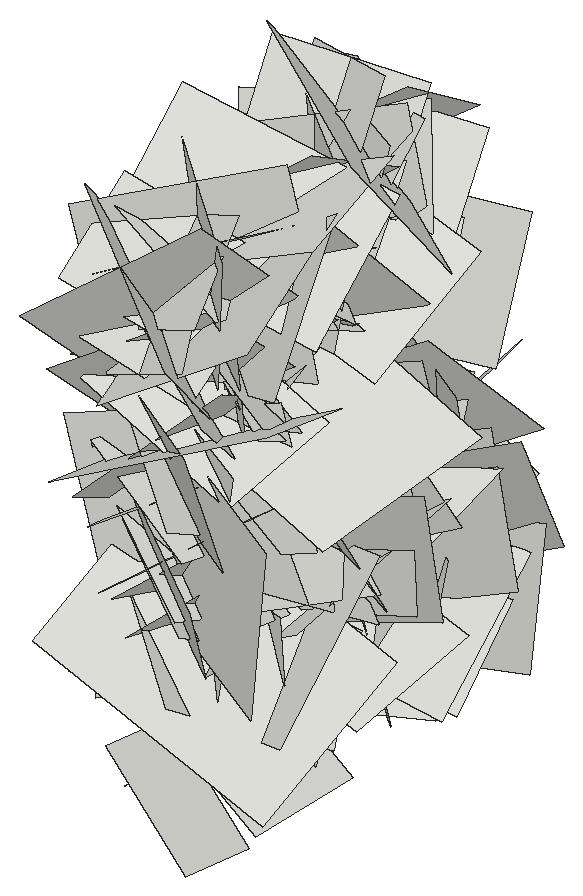
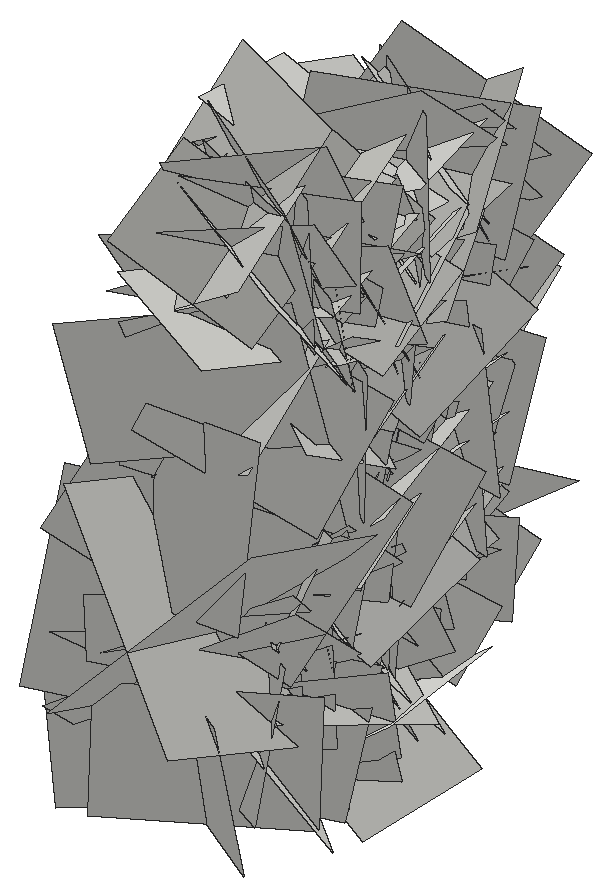
# SketchUp Ruby script. Lengths in inches.
U = 1.inch
M = Sketchup.active_model
def pt(a) = Geom::Point3d.new(a.map { |v| v * U })
def face(e, loops, mat)
  f = e.add_face(loops[0].map { |a| pt(a) })
  loops[1..].each { |l| e.add_face(l.map { |a| pt(a) }).erase! }
  f.material = f.back_material = mat if mat
  f
end
# faces: each face lists its corners as indices into pts; further lists are holes
def faces(e, pts, list, mat = nil) = list.each { |f| face(e, (f[0].is_a?(Array) ? f : [f]).map { |l| l.map { |i| pts[i] } }, mat) }
# xy, xz, yz: faces in a plane at the given z, y or x. An outline is a flat list of corners, or four numbers for a rectangle; further outlines are holes
def ring(l) = l.size == 4 ? [[l[0], l[1]], [l[2], l[1]], [l[2], l[3]], [l[0], l[3]]] : l.each_slice(2).to_a
def flat(e, list, mat, &to3) = list.each { |f| face(e, (f[0].is_a?(Array) ? f : [f]).map { |l| ring(l).map { |u, v| to3.(u, v) } }, mat) }
def xy(e, z, list, mat = nil) = flat(e, list, mat) { |x, y| [x, y, z] }
def xz(e, y, list, mat = nil) = flat(e, list, mat) { |x, z| [x, y, z] }
def yz(e, x, list, mat = nil) = flat(e, list, mat) { |y, z| [x, y, z] }
def lines(e, pts, list) = list.each { |a, b| e.add_line(pt(pts[a]), pt(pts[b])) }
# prism: a flat outline (further loops are holes) pulled along v
def prism(e, loops, v, mat = nil)
  f = face(e, loops, mat); d = Geom::Vector3d.new(v.map { |x| x * U })
  f.pushpull(f.normal.samedirection?(d) ? d.length : -d.length)
end
def box(e, o, s, mat = nil) = prism(e, [[o, [o[0] + s[0], o[1], o[2]], [o[0] + s[0], o[1] + s[1], o[2]], [o[0], o[1] + s[1], o[2]]]], [0, 0, s[2]], mat)
def at(x, y, z, deg = 0) = Geom::Transformation.translation(pt([x, y, z])) * Geom::Transformation.rotation(ORIGIN, Z_AXIS, deg.degrees)
def axes(o, x, y, z) = Geom::Transformation.new([*x, 0, *y, 0, *z, 0, *pt(o).to_a, 1])
def part(name) = M.definitions.add(name)
# library, detail: a bought-in or finely detailed component or shape, given as its bounding box
def library(name, o, s) = part(name).tap { |d| box(d.entities, o, s) }
def detail(e, o, s) = box(e.add_group.entities, o, s)
def put(e, d, t, mat = nil) = e.add_instance(d, t).tap { |i| i.material = mat if mat }
def group(e, t, mat = nil) = e.add_group.tap { |g| g.transformation = t; g.material = mat if mat }.entities
root = M.entities
c1 = part("Component\#6")
p = [[0.01,0,0],[0,3.24,4.54],[4.32,3.24,4.54],[4.33,0,0]]
faces(c1.entities,p,[[0,1,2,3]])
put(root,c1,axes([420.52,193.25,29.42],[-0.0602,0.67546,-0.3863],[-0.10598,-0.39045,-0.66802],[0.81797,-0.00088,-0.11498]))
put(root,c1,axes([420.52,194.71,36.49],[-0.01491,0.71707,-0.22931],[-0.11795,-0.22881,-0.70868],[0.78925,-0.02064,-0.11024]))
put(root,c1,axes([424.49,198.67,35.61],[0.10111,0.59855,0.78971],[-0.15679,0.79307,-0.58323],[-1.03859,-0.06146,0.16492]))
put(root,c1,axes([424.49,206.72,25.52],[0.07134,-1.27871,-0.42932],[0.37284,-0.39835,1.24159],[-1.38032,-0.17369,0.31318]))
put(root,c1,axes([424.49,196.41,37.05],[-0.02372,0.78814,-0.36288],[-0.15491,-0.36124,-0.77556],[-0.90659,0.0411,0.14202]))
put(root,c1,axes([424.49,200.08,36.17],[-0.04967,-0.3024,-0.77978],[-0.15753,-0.76557,0.30582],[-0.87244,0.15545,-0.01082]))
put(root,c1,axes([420.52,194.0625,27.88],[-0.03826,-0.32146,0.75655],[-0.14724,0.74878,0.31153],[0.85881,0.11405,0.08712]))
put(root,c1,axes([420.52,192.62,23.41],[-0.0945,0.05137,0.75973],[0.00531,0.76494,-0.05113],[0.80713,0.00098,0.08928]))
put(root,c1,axes([420.52,194.1,30.97],[-0.07757,0.18705,0.69229],[0.05179,0.69557,-0.18277],[0.75837,-0.02837,0.08329]))
put(root,c1,axes([424.49,192.76,27.5],[0.21382,-0.08753,1.03604],[-0.20559,1.03367,0.1251],[-1.08277,-0.21355,0.18084]))
put(root,c1,axes([420.52,197.11,20.7],[-0.0234,0.20043,0.60552],[0.11848,0.59772,-0.19378],[0.66563,-0.09934,0.05578]))
put(root,c1,axes([424.49,194.12,36.42],[0.16155,0.92195,-0.51802],[-0.06641,-0.51458,-0.93426],[-1.119,0.16364,-0.01934]))
put(root,c1,axes([420.52,192.68,25.51],[0.10584,0.56729,0.32604],[-0.07365,0.33715,-0.56532],[0.68964,-0.05105,-0.11041]))
put(root,c1,axes([424.49,198.72,19.65],[0.06387,-1.04135,0.05905],[0.06023,0.06234,1.04135],[-1.10396,-0.05685,0.06023]))
put(root,c1,axes([424.49,194.92,22.54],[-0.07164,-0.895,0.57486],[0.24411,0.55005,0.88344],[-1.1008,0.18023,0.15849]))
put(root,c1,axes([424.49,200.17,25.9],[-0.12286,-0.34825,-0.84521],[0.12526,-0.85054,0.33424],[-0.96086,-0.06635,0.15165]))
put(root,c1,axes([420.52,196.5,26.6],[-0.00001,0.64808,0.59207],[-0.20568,0.57742,-0.63205],[0.90746,0.13088,-0.14325]))
put(root,c1,axes([424.49,195.45,23.05],[-0.08121,0.42866,0.62692],[-0.16296,0.6083,-0.43472],[-0.78836,-0.1699,0.02528]))
put(root,c1,axes([420.52,201.07,39.9375],[-0.03161,0.68058,-0.41337],[-0.06223,-0.41441,-0.67806],[0.84176,-0.00508,-0.06565]))
put(root,c1,axes([420.52,199.74,34.07],[0.11183,-0.60219,-0.2199],[-0.02555,-0.22643,0.6085],[0.67907,0.09065,0.0591]))
put(root,c1,axes([424.49,195.7,29.31],[0.12944,0.87645,-0.3909],[-0.13192,-0.37627,-0.88251],[-1.00866,0.16168,0.06525]))
put(root,c1,axes([424.49,195.4,26.27],[-0.15303,-0.80886,0.21466],[0.08059,0.20425,0.82078],[-0.8834,0.15875,0.0377]))
put(root,c1,axes([420.52,197.17,21.41],[-0.31691,0.51794,0.91951],[-0.05422,0.94746,-0.55031],[1.11735,0.19287,0.23409]))
put(root,c1,axes([424.49,204.82,25.65],[0.12938,-0.11687,-1.00907],[-0.02351,-1.01639,0.11504],[-1.07651,0.00815,-0.12379]))
put(root,c1,axes([420.52,192.15,39.48],[-0.21361,0.71392,-0.72381],[-0.12034,-0.74908,-0.70723],[1.07091,0.05823,-0.22384]))
put(root,c1,axes([424.49,200.1,34.99],[-0.01875,0.74709,-0.59948],[0.09315,-0.59579,-0.74508],[-1.01106,-0.06874,-0.05753]))
put(root,c1,axes([420.52,198.57,33.25],[-0.09717,0.14422,-0.89801],[-0.11089,-0.89824,-0.13357],[0.95769,-0.08937,-0.10658]))
put(root,c1,axes([424.49,201.91,26.14],[0.02369,0.31708,-0.9382],[0.09459,-0.93526,-0.31396],[-1.04548,-0.07743,-0.04967]))
put(root,c1,axes([424.49,195.16,37.28],[-0.08536,-0.54597,-0.55526],[-0.06407,-0.55215,0.55168],[-0.82294,0.09962,0.01464]))
put(root,c1,axes([420.52,196.95,39.61],[-0.06663,0.78722,-0.39485],[-0.0883,-0.3994,-0.78302],[0.92935,0.01849,-0.10271]))
put(root,c1,axes([420.52,194.17,31.15],[-0.1572,-0.65225,0.62778],[-0.00257,0.63643,0.66066],[0.9596,-0.10514,0.10461]))
put(root,c1,axes([424.49,197.53,26.62],[-0.11622,-0.11144,-0.6986],[-0.08861,-0.69994,0.12478],[-0.74462,0.10068,0.09418]))
put(root,c1,axes([424.49,195.33,34.42],[-0.12228,0.30682,0.85432],[0.19875,0.85067,-0.2802],[-0.94146,0.13973,-0.17012]))
put(root,c1,axes([420.52,195.89,35.57],[-0.03273,-0.74668,0.19464],[0.06894,0.19158,0.74527],[0.81502,-0.04619,-0.05522]))
put(root,c1,axes([420.52,192.38,31.46],[0.05244,0.73173,-0.11131],[0.01157,-0.11227,-0.73318],[0.78447,-0.04726,0.01825]))
put(root,c1,axes([424.49,198.41,25.5],[0.14641,-1.02966,0.26735],[0.10928,0.28128,1.03005],[-1.12233,-0.10694,0.13517]))
put(root,c1,axes([424.49,198.86,35.2],[0.14047,0.16017,0.87964],[-0.13868,0.88315,-0.1411],[-0.93754,-0.10664,0.15267]))
put(root,c1,axes([420.52,193.07,33.95],[0.05953,0.85388,-0.40475],[-0.24794,-0.38029,-0.83472],[0.97048,-0.14953,-0.18843]))
put(root,c1,axes([420.52,201.02,39.48],[-0.13577,0.09163,-0.9618],[-0.05798,-0.96935,-0.08506],[1.02248,-0.0428,-0.13253]))
put(root,c1,axes([420.52,192.92,34.17],[-0.15147,-0.1521,1.01718],[-0.1212,1.02293,0.1369],[1.08344,0.09316,0.15752]))
put(root,c1,axes([424.49,191.375,35.34],[-0.1473,0.40574,0.51918],[-0.07991,0.51733,-0.42447],[-0.69387,-0.14571,-0.06134]))
put(root,c1,axes([424.49,194.18,31.13],[0.04063,-0.16003,0.87853],[0.02386,0.87924,0.15917],[-0.94627,0.0153,0.04174]))
put(root,c1,axes([420.52,202.06,39.63],[-0.00244,-0.36914,-0.6705],[0.07457,-0.66776,0.36739],[0.80789,0.06052,-0.03594]))
put(root,c1,axes([424.49,201.02,32],[0.03236,-0.79816,-0.43551],[0.07074,-0.43262,0.79753],[-0.9612,-0.0587,0.04403]))
put(root,c1,axes([424.49,199.18,25.47],[-0.11604,-0.3767,0.6399],[0.02749,0.64448,0.38383],[-0.78661,0.07809,-0.08099]))
put(root,c1,axes([420.52,199.18,25.47],[0.11604,-0.3767,0.6399],[-0.02749,0.64448,0.38383],[0.78661,0.07809,-0.08099]))
put(root,c1,axes([420.52,201.02,32],[-0.03236,-0.79816,-0.43551],[-0.07074,-0.43262,0.79753],[0.9612,-0.0587,0.04403]))
put(root,c1,axes([424.49,202.06,39.63],[0.00244,-0.36914,-0.6705],[-0.07457,-0.66776,0.36739],[-0.80789,0.06052,-0.03594]))
put(root,c1,axes([420.52,194.18,31.13],[-0.04063,-0.16003,0.87853],[-0.02386,0.87924,0.15917],[0.94627,0.0153,0.04174]))
put(root,c1,axes([420.52,191.375,35.34],[0.1473,0.40574,0.51918],[0.07991,0.51733,-0.42447],[0.69387,-0.14571,-0.06134]))
put(root,c1,axes([424.49,192.92,34.17],[0.15147,-0.1521,1.01718],[0.1212,1.02293,0.1369],[-1.08344,0.09316,0.15752]))
put(root,c1,axes([424.49,201.02,39.48],[0.13577,0.09163,-0.9618],[0.05798,-0.96935,-0.08506],[-1.02248,-0.0428,-0.13253]))
put(root,c1,axes([424.49,193.07,33.95],[-0.05953,0.85388,-0.40475],[0.24794,-0.38029,-0.83472],[-0.97048,-0.14953,-0.18843]))
put(root,c1,axes([420.52,198.86,35.2],[-0.14047,0.16017,0.87964],[0.13868,0.88315,-0.1411],[0.93754,-0.10664,0.15267]))
put(root,c1,axes([420.52,198.41,25.5],[-0.14641,-1.02966,0.26735],[-0.10928,0.28128,1.03005],[1.12233,-0.10694,0.13517]))
put(root,c1,axes([424.49,192.38,31.46],[-0.05244,0.73173,-0.11131],[-0.01157,-0.11227,-0.73318],[-0.78447,-0.04726,0.01825]))
put(root,c1,axes([424.49,195.89,35.57],[0.03273,-0.74668,0.19464],[-0.06894,0.19158,0.74527],[-0.81502,-0.04619,-0.05522]))
put(root,c1,axes([420.52,195.33,34.42],[0.12228,0.30682,0.85432],[-0.19875,0.85067,-0.2802],[0.94146,0.13973,-0.17012]))
put(root,c1,axes([420.52,197.53,26.62],[0.11622,-0.11144,-0.6986],[0.08861,-0.69994,0.12478],[0.74462,0.10068,0.09418]))
put(root,c1,axes([424.49,194.17,31.15],[0.1572,-0.65225,0.62778],[0.00257,0.63643,0.66066],[-0.9596,-0.10514,0.10461]))
put(root,c1,axes([424.49,196.95,39.61],[0.06663,0.78722,-0.39485],[0.0883,-0.3994,-0.78302],[-0.92935,0.01849,-0.10271]))
put(root,c1,axes([420.52,195.16,37.28],[0.08536,-0.54597,-0.55526],[0.06407,-0.55215,0.55168],[0.82294,0.09962,0.01464]))
put(root,c1,axes([420.52,201.91,26.14],[-0.02369,0.31708,-0.9382],[-0.09459,-0.93526,-0.31396],[1.04548,-0.07743,-0.04967]))
put(root,c1,axes([424.49,198.57,33.25],[0.09717,0.14422,-0.89801],[0.11089,-0.89824,-0.13357],[-0.95769,-0.08937,-0.10658]))
put(root,c1,axes([420.52,200.1,34.99],[0.01875,0.74709,-0.59948],[-0.09315,-0.59579,-0.74508],[1.01106,-0.06874,-0.05753]))
put(root,c1,axes([424.49,192.15,39.48],[0.21361,0.71392,-0.72381],[0.12034,-0.74908,-0.70723],[-1.07091,0.05823,-0.22384]))
put(root,c1,axes([420.52,204.82,25.65],[-0.12938,-0.11687,-1.00907],[0.02351,-1.01639,0.11504],[1.07651,0.00815,-0.12379]))
put(root,c1,axes([424.49,197.17,21.41],[0.31691,0.51794,0.91951],[0.05422,0.94746,-0.55031],[-1.11735,0.19287,0.23409]))
put(root,c1,axes([420.52,195.4,26.27],[0.15303,-0.80886,0.21466],[-0.08059,0.20425,0.82078],[0.8834,0.15875,0.0377]))
put(root,c1,axes([420.52,195.7,29.31],[-0.12944,0.87645,-0.3909],[0.13192,-0.37627,-0.88251],[1.00866,0.16168,0.06525]))
put(root,c1,axes([424.49,199.74,34.07],[-0.11183,-0.60219,-0.2199],[0.02555,-0.22643,0.6085],[-0.67907,0.09065,0.0591]))
put(root,c1,axes([424.49,201.07,39.9375],[0.03161,0.68058,-0.41337],[0.06223,-0.41441,-0.67806],[-0.84176,-0.00508,-0.06565]))
put(root,c1,axes([420.52,195.45,23.05],[0.08121,0.42866,0.62692],[0.16296,0.6083,-0.43472],[0.78836,-0.1699,0.02528]))
put(root,c1,axes([424.49,196.5,26.6],[0.00001,0.64808,0.59207],[0.20568,0.57742,-0.63205],[-0.90746,0.13088,-0.14325]))
put(root,c1,axes([420.52,200.17,25.9],[0.12286,-0.34825,-0.84521],[-0.12526,-0.85054,0.33424],[0.96086,-0.06635,0.15165]))
put(root,c1,axes([420.52,194.92,22.54],[0.07164,-0.895,0.57486],[-0.24411,0.55005,0.88344],[1.1008,0.18023,0.15849]))
put(root,c1,axes([420.52,198.72,19.65],[-0.06387,-1.04135,0.05905],[-0.06023,0.06234,1.04135],[1.10396,-0.05685,0.06023]))
put(root,c1,axes([424.49,192.68,25.51],[-0.10584,0.56729,0.32604],[0.07365,0.33715,-0.56532],[-0.68964,-0.05105,-0.11041]))
put(root,c1,axes([420.52,194.12,36.42],[-0.16155,0.92195,-0.51802],[0.06641,-0.51458,-0.93426],[1.119,0.16364,-0.01934]))
put(root,c1,axes([424.49,197.11,20.7],[0.0234,0.20043,0.60552],[-0.11848,0.59772,-0.19378],[-0.66563,-0.09934,0.05578]))
put(root,c1,axes([420.52,192.76,27.5],[-0.21382,-0.08753,1.03604],[0.20559,1.03367,0.1251],[1.08277,-0.21355,0.18084]))
put(root,c1,axes([424.49,194.1,30.97],[0.07757,0.18705,0.69229],[-0.05179,0.69557,-0.18277],[-0.75837,-0.02837,0.08329]))
put(root,c1,axes([424.49,192.62,23.41],[0.0945,0.05137,0.75973],[-0.00531,0.76494,-0.05113],[-0.80713,0.00098,0.08928]))
put(root,c1,axes([424.49,194.0625,27.88],[0.03826,-0.32146,0.75655],[0.14724,0.74878,0.31153],[-0.85881,0.11405,0.08712]))
put(root,c1,axes([420.52,200.08,36.17],[0.04967,-0.3024,-0.77978],[0.15753,-0.76557,0.30582],[0.87244,0.15545,-0.01082]))
put(root,c1,axes([420.52,196.41,37.05],[0.02372,0.78814,-0.36288],[0.15491,-0.36124,-0.77556],[0.90659,0.0411,0.14202]))
put(root,c1,axes([420.52,206.72,25.52],[-0.07134,-1.27871,-0.42932],[-0.37284,-0.39835,1.24159],[1.38032,-0.17369,0.31318]))
put(root,c1,axes([420.52,198.67,35.61],[-0.10111,0.59855,0.78971],[0.15679,0.79307,-0.58323],[1.03859,-0.06146,0.16492]))
put(root,c1,axes([424.49,194.71,36.49],[0.01491,0.71707,-0.22931],[0.11795,-0.22881,-0.70868],[-0.78925,-0.02064,-0.11024]))
put(root,c1,axes([424.49,193.25,29.42],[0.0602,0.67546,-0.3863],[0.10598,-0.39045,-0.66802],[-0.81797,-0.00088,-0.11498]))
put(root,c1,axes([424.49,198.68,37.125],[-0.06347,0.58127,-0.24952],[0.07215,-0.24326,-0.58302],[-0.66662,-0.08167,-0.03935]))
put(root,c1,axes([420.52,195.125,35.61],[0.03117,0.92717,-0.40656],[-0.02653,-0.40594,-0.92757],[1.07281,-0.03698,-0.01113]))
put(root,c1,axes([424.49,200.57,36.04],[0.10099,0.61602,0.17436],[-0.1325,0.19079,-0.60575],[-0.66557,0.05549,0.14705]))
put(root,c1,axes([420.52,197.34,38.49],[0.22162,0.66132,-0.53694],[-0.02723,-0.54773,-0.68462],[0.90256,-0.17891,0.1112]))
put(root,c1,axes([420.52,198.8,27.02],[-0.0226,-0.2767,0.96977],[0.06915,0.96758,0.27751],[1.06674,-0.06859,0.00256]))
put(root,c1,axes([420.52,193.58,33.2],[0.1306,0.22319,-0.86205],[0.05382,-0.87061,-0.21815],[0.94237,0.01879,0.13193]))
put(root,c1,axes([420.52,197.85,24.73],[-0.35143,-0.52734,1.13432],[0.18025,1.14359,0.58135],[1.31365,-0.29799,0.22369]))
put(root,c1,axes([424.49,196.3,29.33],[0.09147,0.43894,-0.4809],[-0.05464,-0.47898,-0.44644],[-0.688,0.09639,-0.02848]))
put(root,c1,axes([424.49,192.39,25.48],[0.15082,-0.34829,0.66058],[0.01541,0.67363,0.35204],[-0.79143,-0.05326,0.13274]))
put(root,c1,axes([420.52,199.8,22.82],[-0.00598,0.07204,1.08492],[-0.02761,1.08461,-0.07215],[1.15221,0.02636,0.0039]))
put(root,c1,axes([424.49,194.26,19.42],[0.05867,-0.70774,0.13488],[0.12622,0.14241,0.69835],[-0.75321,-0.03127,0.12754]))
put(root,c1,axes([420.52,196.22,30.25],[-0.08073,-0.93811,0.99109],[-0.27356,0.98462,0.91216],[1.42044,0.13631,0.232]))
put(root,c1,axes([420.52,191.97,33.56],[0.08688,0.89449,0.25558],[0.12211,0.24484,-0.89383],[0.97851,-0.10998,0.08885]))
put(root,c1,axes([420.52,197.83,24.35],[-0.09568,0.96283,0.81475],[-0.1112,0.80827,-0.9668],[1.33234,0.1366,-0.02218]))
put(root,c1,axes([420.52,199.05,27.98],[0.08019,0.19915,0.92966],[0.13728,0.92174,-0.20799],[0.9984,-0.14274,-0.04607]))
put(root,c1,axes([420.52,202.95,33.21],[-0.17447,0.42234,-1.07867],[0.17991,-1.06896,-0.44444],[1.21466,0.21899,-0.08911]))
put(root,c1,axes([420.52,201.66,25.46],[-0.21728,-0.88431,0.94199],[0.03627,0.94972,0.89901],[1.36907,-0.16551,0.12568]))
put(root,c1,axes([420.52,195.04,27.27],[0.2131,0.57774,0.71728],[0.02179,0.73117,-0.59469],[0.97604,-0.14247,-0.14333]))
put(root,c1,axes([420.52,197.22,25.56],[0.17769,-0.12121,-0.94504],[0.07151,-0.95564,0.13453],[1.00742,0.08922,0.15714]))
put(root,c1,axes([420.52,192.77,37.47],[-0.01566,0.85002,0.74451],[0.07038,0.74394,-0.84805],[1.19569,-0.03266,0.05967]))
put(root,c1,axes([424.49,203.75,35.72],[0.12855,-0.35471,-0.52952],[0.05195,-0.53223,0.36775],[-0.67359,-0.10874,-0.07269]))
put(root,c1,axes([420.52,202.23,24.6],[-0.19755,-1.2824,-0.48224],[-0.04087,-0.48158,1.29554],[1.4517,-0.18807,-0.02915]))
put(root,c1,axes([420.52,200.11,31.93],[0.08158,0.26048,1.04137],[0.05734,1.04178,-0.26458],[1.13642,-0.07126,-0.06141]))
put(root,c1,axes([420.52,198.78,35.93],[0.06513,-0.64723,-0.92238],[0.00055,-0.92374,0.64822],[1.19442,0.03572,0.05]))
put(root,c1,axes([420.52,196.35,35.86],[0.06555,0.97369,0.5362],[0.0688,0.53295,-0.97527],[1.17625,-0.08544,0.02716]))
put(root,c1,axes([420.52,195.34,33.06],[0.01901,1.14103,-0.72029],[-0.19621,-0.71146,-1.13165],[1.41679,-0.11384,-0.14706]))
put(root,c1,axes([420.52,197.73,24.08],[0.06299,0.80841,0.87356],[-0.01823,0.87514,-0.8087],[1.26151,-0.02772,-0.0553]))
put(root,c1,axes([420.52,194.3,32.47],[-0.23408,0.14056,-1.33491],[0.22407,-1.33233,-0.17526],[1.40507,0.23589,-0.19445]))
put(root,c1,axes([420.52,196.04,25.17],[0.02819,1.07686,0.22249],[0.25409,0.21152,-1.05244],[1.13755,-0.07393,0.22957]))
put(root,c1,axes([420.52,193.85,32.27],[0.12737,1.17977,-0.33684],[-0.1012,-0.32843,-1.18439],[1.29659,-0.14153,-0.05935]))
put(root,c1,axes([420.52,198.24,37.08],[0.15669,-0.99926,-0.19378],[0.22295,-0.1616,0.99377],[1.05566,0.18244,-0.18112]))
put(root,c1,axes([420.52,197.21,31.46],[0.04455,0.58157,-0.95839],[0.2239,-0.94599,-0.56478],[1.16701,0.1593,0.14494]))
put(root,c1,axes([420.52,200.75,21.625],[0.14431,-0.01788,1.13958],[0.06693,1.14604,0.01044],[1.20625,-0.06145,-0.13692]))
put(root,c1,axes([420.52,198.29,23.22],[0.04433,-0.32511,1.32538],[-0.126,1.3201,0.32757],[1.44106,0.12543,-0.01213]))
put(root,c1,axes([420.52,196.35,30.1],[0.25467,1.00338,0.64071],[-0.12934,0.67094,-1.00496],[1.25528,-0.13443,-0.23354]))
put(root,c1,axes([420.52,199.72,26.12],[-0.08735,-0.8928,-1.02237],[0.07635,-1.02569,0.88989],[1.43674,0.00023,-0.10945]))
put(root,c1,axes([420.52,196.54,35.06],[0.17609,-1.11494,-0.45613],[-0.00034,-0.46049,1.12547],[1.27691,0.15363,0.0632]))
put(root,c1,axes([420.52,189.88,26.35],[0.12674,1.17916,0.69894],[-0.07675,0.70605,-1.17877],[1.45096,-0.06565,-0.1234]))
put(root,c1,axes([420.52,194.52,25.48],[0.11423,-0.20624,1.26777],[0.06819,1.2715,0.20138],[1.3598,-0.04643,-0.1166]))
put(root,c1,axes([420.52,193.84,30.46],[0.25587,-1.06575,0.3461],[0.15582,0.3811,1.07099],[1.17751,0.18115,-0.21693]))
put(root,c1,axes([420.52,199.97,41.09],[0.2759,0.65189,-0.94787],[0.07756,-0.97924,-0.65337],[1.21695,-0.08538,0.25653]))
put(root,c1,axes([420.52,200.57,23.13],[0.2198,-0.69796,1.13548],[-0.0671,1.14269,0.71395],[1.41122,0.16304,-0.1429]))
put(root,c1,axes([420.52,195.625,24.52],[0.22176,-0.47224,1.18941],[0.10161,1.2076,0.46259],[1.3527,-0.0133,-0.22974]))
put(root,c1,axes([420.52,193.54,33.12],[0.22081,1.30446,0.31828],[0.37279,0.25784,-1.28691],[1.3736,-0.27967,0.29809]))
